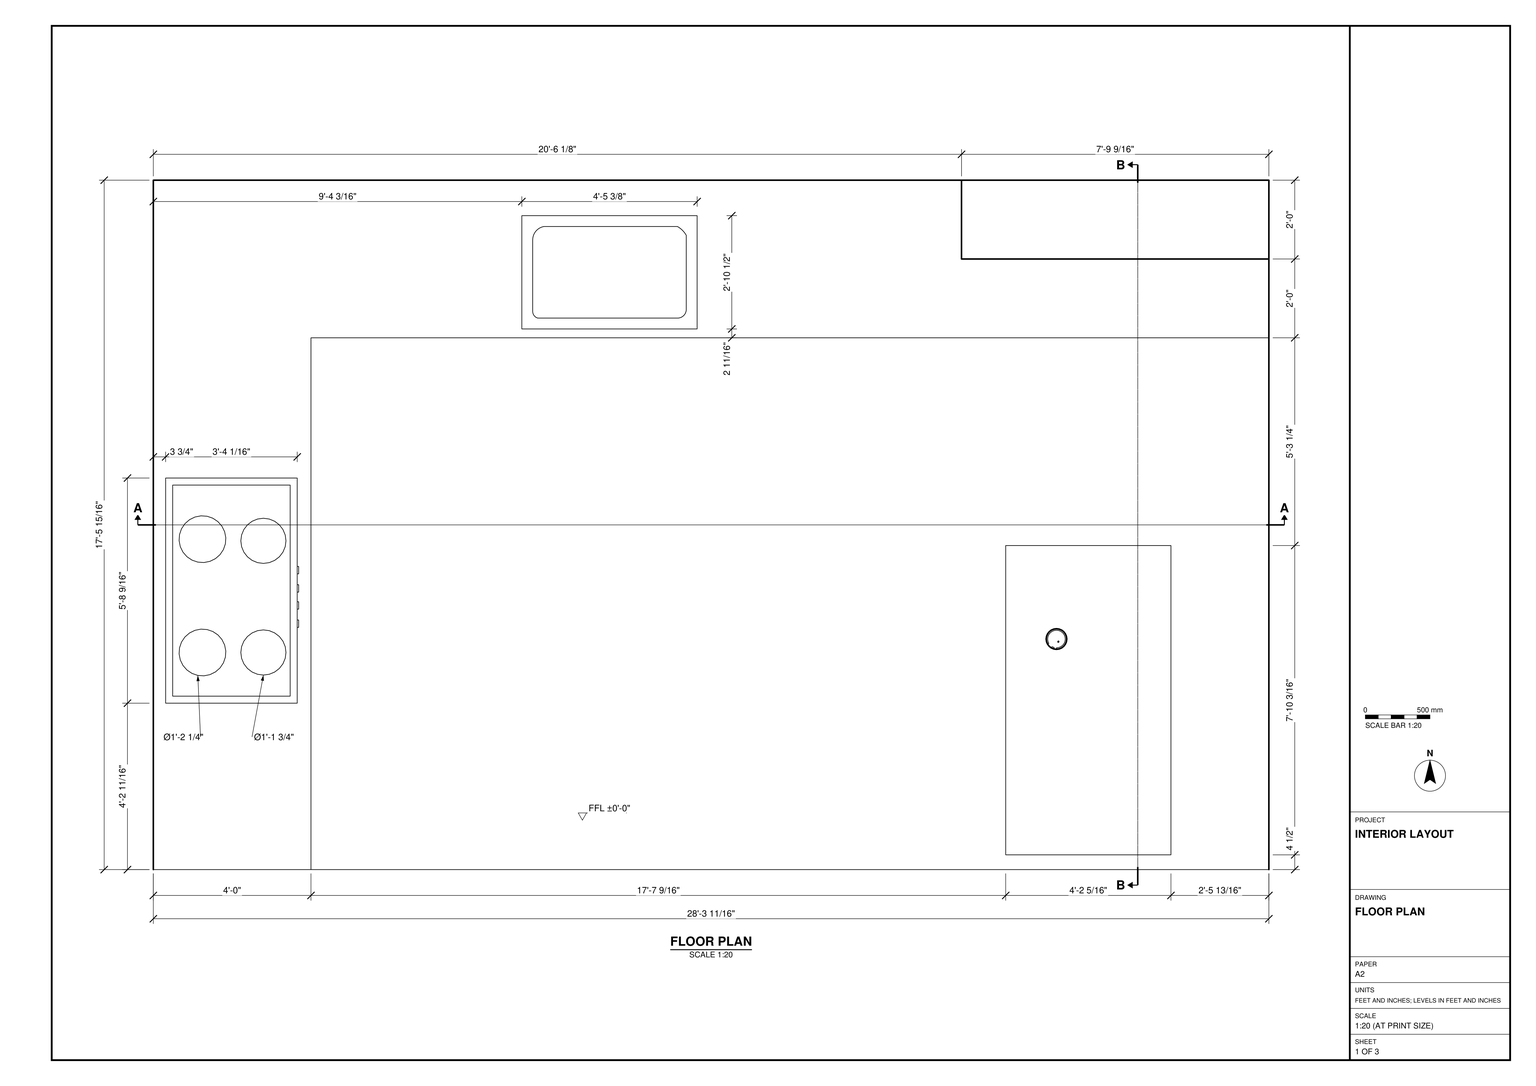
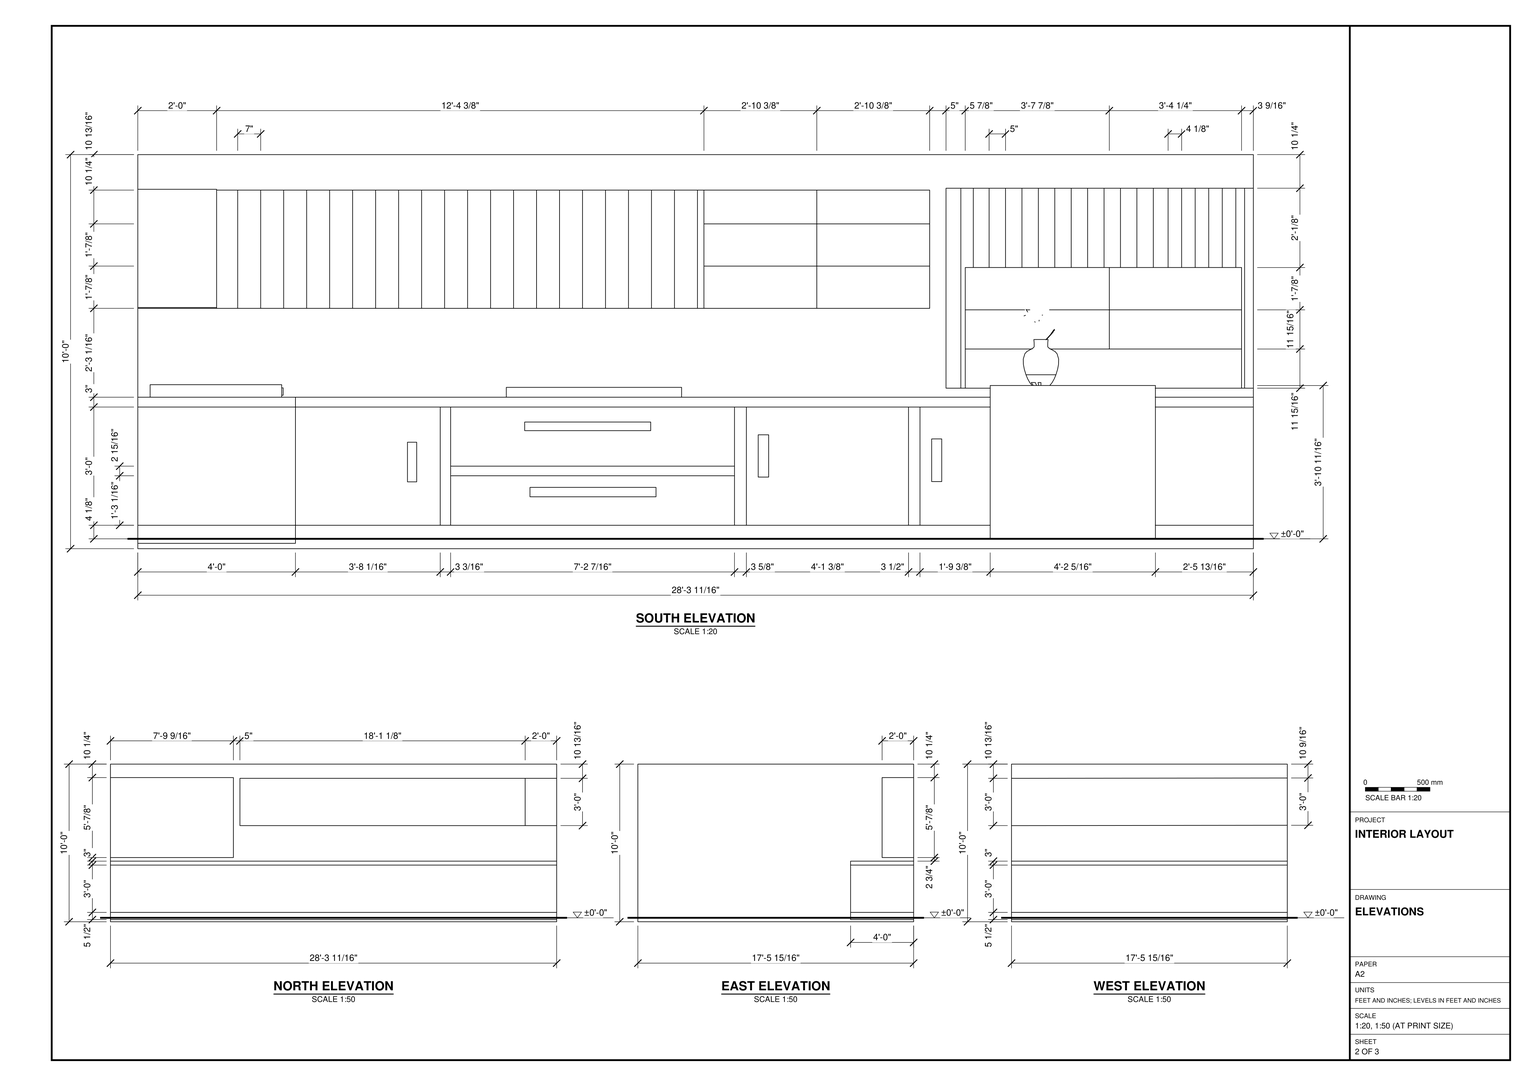
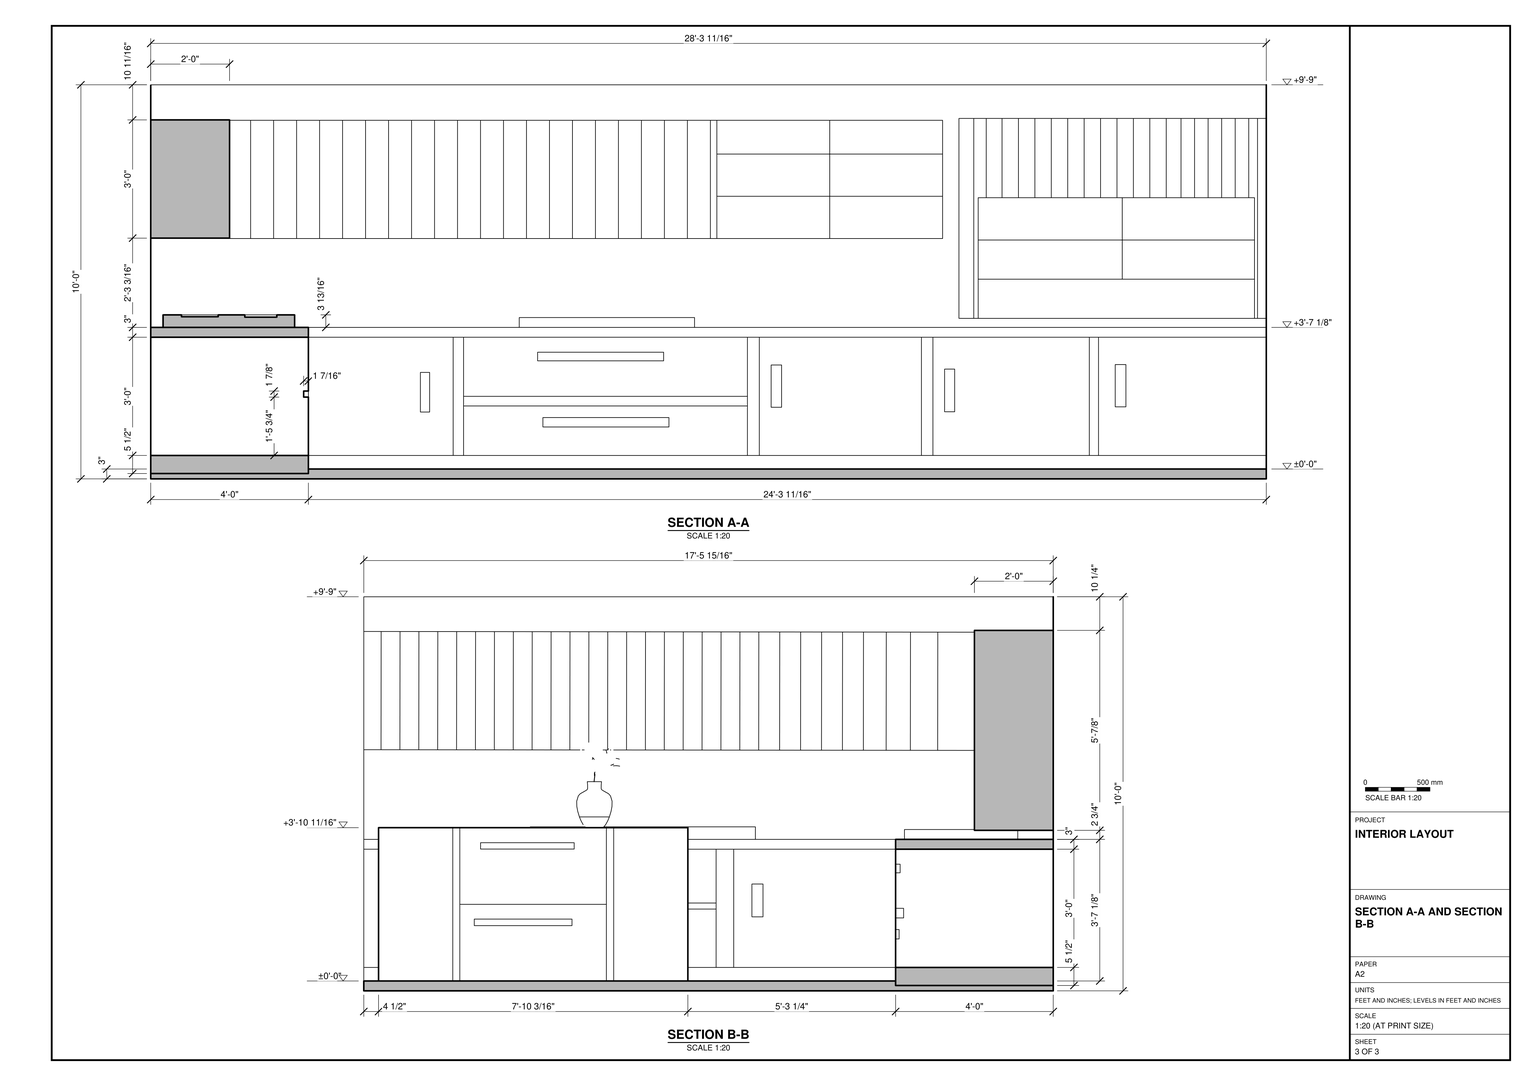
Build the kitchen interior in SketchUp from task_files/diagram_01.pdf. Work in feet and inches. The overall size is 28'-3 11/16" along X, 17'-5 15/16" along Y and 10'-0" vertically. Use the single finished-floor level of ±0'-0". Model the floor slab and the wall extents and thicknesses shown in the elevations and sections.

Use the floor plan to lay out the L-shaped counter along the top and left edges of the room. Place the sink in the long run and the cooktop on the left return. Use section A-A to set the worktop, plinth and cabinet heights. Match the arrangement of base cabinet doors, wide drawers and pulls. Above the worktop, distinguish the long band of narrow vertical panels from the horizontally divided cabinet bays, including the deeper hanging unit at the right end of the south elevation.

Set out the freestanding island from the bottom and right edges of the plan, with its long side parallel to the cooktop return. Use section B-B for its top height and drawer arrangement. Place a vase on the island as shown. Decor and loose items may be any suitable library components, for example from 3D Warehouse.

Keep shell elements such as walls and the floor slab in separate groups or components, group each furniture or joinery piece separately, and use components for repeated parts. Save one SketchUp model as output_files/l_shaped_kitchen_with_a_freestanding_storage_island.skp.

# SketchUp Ruby script. Lengths in inches.
U = 1.inch
M = Sketchup.active_model
def pt(a) = Geom::Point3d.new(a.map { |v| v * U })
def face(e, loops, mat)
  f = e.add_face(loops[0].map { |a| pt(a) })
  loops[1..].each { |l| e.add_face(l.map { |a| pt(a) }).erase! }
  f.material = f.back_material = mat if mat
  f
end
# faces: each face lists its corners as indices into pts; further lists are holes
def faces(e, pts, list, mat = nil) = list.each { |f| face(e, (f[0].is_a?(Array) ? f : [f]).map { |l| l.map { |i| pts[i] } }, mat) }
# xy, xz, yz: faces in a plane at the given z, y or x. An outline is a flat list of corners, or four numbers for a rectangle; further outlines are holes
def ring(l) = l.size == 4 ? [[l[0], l[1]], [l[2], l[1]], [l[2], l[3]], [l[0], l[3]]] : l.each_slice(2).to_a
def flat(e, list, mat, &to3) = list.each { |f| face(e, (f[0].is_a?(Array) ? f : [f]).map { |l| ring(l).map { |u, v| to3.(u, v) } }, mat) }
def xy(e, z, list, mat = nil) = flat(e, list, mat) { |x, y| [x, y, z] }
def xz(e, y, list, mat = nil) = flat(e, list, mat) { |x, z| [x, y, z] }
def yz(e, x, list, mat = nil) = flat(e, list, mat) { |y, z| [x, y, z] }
def lines(e, pts, list) = list.each { |a, b| e.add_line(pt(pts[a]), pt(pts[b])) }
# prism: a flat outline (further loops are holes) pulled along v
def prism(e, loops, v, mat = nil)
  f = face(e, loops, mat); d = Geom::Vector3d.new(v.map { |x| x * U })
  f.pushpull(f.normal.samedirection?(d) ? d.length : -d.length)
end
def box(e, o, s, mat = nil) = prism(e, [[o, [o[0] + s[0], o[1], o[2]], [o[0] + s[0], o[1] + s[1], o[2]], [o[0], o[1] + s[1], o[2]]]], [0, 0, s[2]], mat)
def at(x, y, z, deg = 0) = Geom::Transformation.translation(pt([x, y, z])) * Geom::Transformation.rotation(ORIGIN, Z_AXIS, deg.degrees)
def axes(o, x, y, z) = Geom::Transformation.new([*x, 0, *y, 0, *z, 0, *pt(o).to_a, 1])
def part(name) = M.definitions.add(name)
# library, detail: a bought-in or finely detailed component or shape, given as its bounding box
def library(name, o, s) = part(name).tap { |d| box(d.entities, o, s) }
def detail(e, o, s) = box(e.add_group.entities, o, s)
def put(e, d, t, mat = nil) = e.add_instance(d, t).tap { |i| i.material = mat if mat }
def group(e, t, mat = nil) = e.add_group.tap { |g| g.transformation = t; g.material = mat if mat }.entities
root = M.entities
M.materials.add("[Blacktop New]").color = [30, 30, 30]
M.materials.add("[Blacktop Old 01]").color = [132, 136, 139]
M.materials.add("[Blinds Weave]").color = [141, 91, 25]
M.materials.add("[Concrete Tile]").color = [203, 190, 164]
M.materials.add("[Tile Ceramic Natural]").color = [216, 206, 153]
M.materials.add("[Tile Limestone Multi]").color = [199, 173, 118]
M.materials.add("[Translucent Glass Block Dark]").color = [124, 124, 121]
M.materials["[Translucent Glass Block Dark]"].alpha = 0.8
M.materials.add("[Translucent Glass Blue]").color = [100, 149, 237]
M.materials["[Translucent Glass Blue]"].alpha = 0.5
c1 = library("Flower+vase",[-27.04,-0.0625,0],[7.8,7.11,11.89])
xy(root,0,[[0,0,339.6875,209.9375]])
xy(root,1.625,[[0,0,0,209.9375,339.6875,209.9375,339.6875,161.9375,48,161.9375,48,0]])
xy(root,3,[[[48,0,339.6875,161.9375],[259.55,4.49,309.86,98.68]],[259.55,4.49,309.86,98.68]],"[Tile Ceramic Natural]")
xy(root,7.125,[[0,0,0,209.9375,339.6875,209.9375,339.6875,161.9375,48,161.9375,48,0]])
xy(root,15.8,[[119.41,161.9375,157.79,163]],"[Blacktop Old 01]")
xy(root,17.51,[[46.625,57.29,48,85.85]],"[Blacktop Old 01]")
xy(root,18.67,[[119.41,161.9375,157.79,163]])
xy(root,19.85,[[259.55,33.64,260.43,63.39]],"[Tile Ceramic Natural]")
xy(root,20.58,[[46.625,57.29,48,85.85]])
xy(root,21.85,[[259.55,33.64,260.43,63.39]],"[Tile Ceramic Natural]")
xy(root,22.2,[[95.26,161.9375,181.69,164.375]],"[Blacktop New]")
xy(root,24.9,[[46.5625,41.5,48,107.28]],"[Blacktop New]")
xy(root,25.125,[[95.26,161.9375,181.69,164.375]])
xy(root,26.74,[[46.5625,41.5,48,107.28]])
xy(root,34.63,[[46.875,55.84,48,85.21]],"[Blacktop New]")
xy(root,35.94,[[117.8,161.9375,156.18,163.3125]],"[Blacktop New]")
xy(root,38.38,[[46.875,55.84,48,85.21]])
xy(root,38.57,[[117.8,161.9375,156.18,163.3125]])
xy(root,43.125,[[0,0,0,209.9375,339.6875,209.9375,339.6875,161.9375,48,161.9375,48,0]])
xy(root,43.17,[[259.55,35.5625,260.74,64.0625]],"[Tile Ceramic Natural]")
xy(root,45.11,[[259.55,35.5625,260.74,64.0625]],"[Tile Ceramic Natural]")
xy(root,46.125,[[[0,0,48,0,48,161.9375,339.6875,161.9375,339.6875,209.9375,0,209.9375],[3.75,50.67,43.8125,119.24],[112.21,164.64,165.59,199.14]],[3.75,50.67,43.8125,119.24],[[112.21,164.64,165.59,199.14],[117.08,167.94,159.625,167.94,159.97,167.96,160.3125,168.03,160.64,168.14,160.95,168.3,161.24,168.49,161.5,168.72,161.73,168.98,161.93,169.27,162.08,169.58,162.19,169.91,162.26,170.25,162.28,170.6,162.28,193.14,162.12,193.42,161.94,193.6875,161.75,193.95,161.55,194.2,161.34,194.4375,161.12,194.67,160.89,194.89,160.65,195.1,160.4,195.3,160.14,195.49,159.87,195.67,159.59,195.83,118.91,195.83,118.45,195.72,118,195.55,117.57,195.33,117.17,195.07,116.8,194.76,116.48,194.41,116.19,194.02,115.95,193.61,115.76,193.17,115.63,192.71,115.54,192.24,115.52,191.76,115.52,169.98,115.53,169.75,115.57,169.53,115.63,169.31,115.71,169.09,115.82,168.89,115.95,168.7,116.1,168.53,116.27,168.37,116.45,168.23,116.65,168.11,116.86,168.01]]],"[Concrete Tile]")
xy(root,48.875,[[246.09,185.9375,339.6875,209.9375]])
xy(root,49,[[33.51,59.24,35.29,59.48,36.95,60.16,38.375,61.26,39.47,62.68,40.15,64.34,40.39,66.12,40.15,67.9,39.47,69.56,38.375,70.98,36.95,72.07,35.29,72.76,33.51,72.99,31.73,72.76,30.08,72.07,28.65,70.98,27.56,69.56,26.875,67.9,26.64,66.12,26.875,64.34,27.56,62.68,28.65,61.26,30.08,60.16,31.73,59.48]],"[Concrete Tile]")
xy(root,49.125,[[[112.21,164.64,165.59,199.14],[117.08,167.94,116.86,168.01,116.65,168.11,116.45,168.23,116.27,168.37,116.1,168.53,115.95,168.7,115.82,168.89,115.71,169.09,115.63,169.31,115.57,169.53,115.53,169.75,115.52,169.98,115.52,191.76,115.54,192.24,115.63,192.71,115.76,193.17,115.95,193.61,116.19,194.02,116.48,194.41,116.8,194.76,117.17,195.07,117.57,195.33,118,195.55,118.45,195.72,118.91,195.83,159.59,195.83,159.87,195.67,160.14,195.49,160.4,195.3,160.65,195.1,160.89,194.89,161.12,194.67,161.34,194.4375,161.55,194.2,161.75,193.95,161.94,193.6875,162.12,193.42,162.28,193.14,162.28,170.6,162.26,170.25,162.19,169.91,162.08,169.58,161.93,169.27,161.73,168.98,161.5,168.72,161.24,168.49,160.95,168.3,160.64,168.14,160.3125,168.03,159.97,167.96,159.625,167.94]]],"[Concrete Tile]")
xy(root,49.25,[[33.51,93.24,35.29,93.48,36.95,94.16,38.375,95.26,39.47,96.68,40.15,98.34,40.39,100.12,40.15,101.9,39.47,103.56,38.375,104.98,36.95,106.07,35.29,106.76,33.51,106.99,31.73,106.76,30.08,106.07,28.65,104.98,27.56,103.56,26.875,101.9,26.64,100.12,26.875,98.34,27.56,96.68,28.65,95.26,30.08,94.16,31.73,93.48]],"[Concrete Tile]")
xy(root,49.375,[[15.41,59.01,17.23,59.37,18.9,60.1875,20.3,61.41,21.34,62.95,21.94,64.71,22.07,66.57,21.71,68.39,20.89,70.0625,19.67,71.47,18.12,72.5,16.36,73.1,14.5,73.23,12.68,72.87,11.01,72.05,9.61,70.83,8.57,69.28,7.97,67.52,7.85,65.67,8.2,63.84,9.02,62.17,10.25,60.77,11.79,59.73,13.55,59.13],[15.41,93.51,17.23,93.87,18.9,94.6875,20.3,95.91,21.34,97.45,21.94,99.21,22.07,101.07,21.71,102.89,20.89,104.5625,19.67,105.97,18.12,107,16.36,107.6,14.5,107.73,12.68,107.37,11.01,106.55,9.61,105.33,8.57,103.78,7.97,102.02,7.85,100.17,8.2,98.34,9.02,96.67,10.25,95.27,11.79,94.23,13.55,93.63]],"[Concrete Tile]")
xy(root,49.6875,[[259.55,4.49,309.86,98.68]],"[Tile Ceramic Natural]")
xy(root,49.9375,[[[5.89,52.81,41.67,117.09],[15.41,59.01,13.55,59.13,11.79,59.73,10.25,60.77,9.02,62.17,8.2,63.84,7.85,65.67,7.97,67.52,8.57,69.28,9.61,70.83,11.01,72.05,12.68,72.87,14.5,73.23,16.36,73.1,18.12,72.5,19.67,71.47,20.89,70.0625,21.71,68.39,22.07,66.57,21.94,64.71,21.34,62.95,20.3,61.41,18.9,60.1875,17.23,59.37],[15.41,93.51,13.55,93.63,11.79,94.23,10.25,95.27,9.02,96.67,8.2,98.34,7.85,100.17,7.97,102.02,8.57,103.78,9.61,105.33,11.01,106.55,12.68,107.37,14.5,107.73,16.36,107.6,18.12,107,19.67,105.97,20.89,104.5625,21.71,102.89,22.07,101.07,21.94,99.21,21.34,97.45,20.3,95.91,18.9,94.6875,17.23,93.87],[33.51,59.24,31.73,59.48,30.08,60.16,28.65,61.26,27.56,62.68,26.875,64.34,26.64,66.12,26.875,67.9,27.56,69.56,28.65,70.98,30.08,72.07,31.73,72.76,33.51,72.99,35.29,72.76,36.95,72.07,38.375,70.98,39.47,69.56,40.15,67.9,40.39,66.12,40.15,64.34,39.47,62.68,38.375,61.26,36.95,60.16,35.29,59.48],[33.51,93.24,31.73,93.48,30.08,94.16,28.65,95.26,27.56,96.68,26.875,98.34,26.64,100.12,26.875,101.9,27.56,103.56,28.65,104.98,30.08,106.07,31.73,106.76,33.51,106.99,35.29,106.76,36.95,106.07,38.375,104.98,39.47,103.56,40.15,101.9,40.39,100.12,40.15,98.34,39.47,96.68,38.375,95.26,36.95,94.16,35.29,93.48]]],"[Blacktop New]")
xy(root,49.9375,[[[3.75,50.67,43.8125,119.24],[5.89,52.81,41.67,117.09]]],"[Concrete Tile]")
xy(root,73.1875,[[24,185.9375,241.125,209.9375]],"[Blinds Weave]")
xy(root,109.1875,[[24,185.9375,241.125,209.9375]],"[Blinds Weave]")
xy(root,109.76,[[246.09,185.9375,339.6875,209.9375]],"[Blinds Weave]")
xz(root,0,[[0,73.4375,24,109.4375]],"[Blinds Weave]")
xz(root,0,[[0,43.125,48,46.125]],"[Concrete Tile]")
xz(root,0,[[0,0,339.6875,0,339.6875,3,48,3,48,1.625,0,1.625]],"[Tile Ceramic Natural]")
xz(root,0,[[0,1.625,48,7.125],[0,7.125,48,43.125]],"[Tile Limestone Multi]")
xz(root,4.49,[[259.55,3,309.86,49.6875]],"[Tile Ceramic Natural]")
xz(root,33.64,[[259.55,19.85,260.43,21.85]],"[Tile Ceramic Natural]")
xz(root,35.5625,[[259.55,43.17,260.74,45.11]],"[Tile Ceramic Natural]")
xz(root,41.5,[[46.5625,24.9,48,26.74]])
xz(root,50.67,[[3.75,46.125,43.8125,49.9375]],"[Concrete Tile]")
xz(root,55.84,[[46.875,34.63,48,38.38]])
xz(root,57.29,[[46.625,17.51,48,20.58]])
xz(root,63.39,[[259.55,19.85,260.43,21.85]],"[Tile Ceramic Natural]")
xz(root,64.0625,[[259.55,43.17,260.74,45.11]],"[Tile Ceramic Natural]")
xz(root,85.21,[[46.875,34.63,48,38.38]],"[Blacktop New]")
xz(root,85.85,[[46.625,17.51,48,20.58]],"[Blacktop Old 01]")
xz(root,98.68,[[259.55,3,309.86,49.6875]],"[Tile Ceramic Natural]")
xz(root,107.28,[[46.5625,24.9,48,26.74]],"[Blacktop Old 01]")
xz(root,119.24,[[3.75,46.125,43.8125,49.9375]],"[Concrete Tile]")
xz(root,161.9375,[[48,1.625,339.6875,3]])
xz(root,161.9375,[[82.11,20.35,84.92,32.42],[241.73,20.43,244.79,33.43],[188.91,21.8,192.1,34.68],[293.6875,21.93,296.9375,34.81]],"[Blacktop Old 01]")
xz(root,161.9375,[[48,43.125,339.6875,46.125]],"[Concrete Tile]")
xz(root,161.9375,[[48,3,339.6875,7.125],[[48,7.125,92.09,43.125],[82.11,20.35,84.92,32.42]],[92.09,7.125,95.26,43.125],[[95.26,7.125,181.69,22.2],[119.41,15.8,157.79,18.67]],[181.69,7.125,185.3125,43.125],
  [[185.3125,7.125,234.68,43.125],[188.91,21.8,192.1,34.68]],[234.68,7.125,238.18,43.125],[[238.18,7.125,285.8,43.125],[241.73,20.43,244.79,33.43]],[285.8,7.125,288.6,43.125],[[288.6,7.125,339.6875,43.125],[293.6875,21.93,296.9375,34.81]],
  [[95.26,25.125,181.69,43.125],[117.8,35.94,156.18,38.57]]],"[Tile Limestone Multi]")
xz(root,163,[[119.41,15.8,157.79,18.67]],"[Blacktop Old 01]")
xz(root,163.3125,[[117.8,35.94,156.18,38.57]],"[Blacktop New]")
xz(root,164.375,[[95.26,22.2,181.69,25.125]],"[Blacktop New]")
xz(root,164.64,[[112.21,46.125,165.59,49.125]],"[Concrete Tile]")
xz(root,167.94,[[117.08,46.125,159.625,49.125]],"[Concrete Tile]")
xz(root,185.9375,[[246.09,48.875,250.61,109.76],[250.61,48.875,251.96,48.875,251.96,85.62,254.41,85.62,254.41,109.76,250.61,109.76],[336.09,48.875,337.02,48.875,337.02,109.76,334.35,109.76,334.35,85.62,336.09,85.62],[337.02,48.875,339.6875,109.76],[24,73.1875,172.38,109.1875],
  [254.41,85.62,259.22,109.76],[259.22,85.62,264.22,109.76],[264.22,85.62,269.22,109.76],[269.22,85.62,274.22,109.76],[274.22,85.62,279.22,109.76],
  [279.22,85.62,284.22,109.76],[284.22,85.62,289.22,109.76],[289.22,85.62,294.22,109.76],[294.22,85.62,299.22,109.76],[299.22,85.62,304.22,109.76],
  [304.22,85.62,309.22,109.76],[309.22,85.62,313.72,109.76],[313.72,85.62,317.85,109.76],[317.85,85.62,321.97,109.76],[321.97,85.62,326.1,109.76],
  [326.1,85.62,330.22,109.76],[330.22,85.62,334.35,109.76]],"[Blinds Weave]")
xz(root,185.9375,[[251.96,48.875,336.09,60.8]],"[Translucent Glass Block Dark]")
xz(root,185.9375,[[251.96,60.8,295.82,72.73],[295.82,60.8,336.09,72.73],[251.96,72.73,295.82,85.62],[295.82,72.73,336.09,85.62],[172.38,73.1875,206.75,86.05],
  [206.75,73.1875,241.125,86.05],[172.38,86.05,206.75,98.91],[206.75,86.05,241.125,98.91],[172.38,98.91,206.75,109.1875],[206.75,98.91,241.125,109.1875]],"[Translucent Glass Blue]")
xz(root,195.83,[[118.91,46.125,159.59,49.125]],"[Concrete Tile]")
xz(root,199.14,[[112.21,46.125,165.59,49.125]],"[Concrete Tile]")
xz(root,209.9375,[[0,0,339.6875,1.625],[0,1.625,339.6875,7.125],[0,7.125,339.6875,43.125],[0,43.125,339.6875,46.125],[0,46.125,0,73.1875,241.125,73.1875,241.125,109.1875,0,109.1875,0,120,339.6875,120,339.6875,109.76,246.09,109.76,246.09,48.875,339.6875,48.875,339.6875,46.125],
  [246.09,48.875,339.6875,109.76],[0,73.1875,24,109.1875],[24,73.1875,241.125,109.1875]],"[Blacktop Old 01]")
yz(root,0,[[0,0,209.9375,1.625]])
yz(root,0,[[0,1.625,209.9375,7.125],[0,7.125,209.9375,43.125],[0,43.125,209.9375,46.125],[0,46.125,0,73.4375,209.9375,73.1875,209.9375,46.125],[209.9375,73.1875,0,73.4375,0,109.4375,209.9375,109.1875],
  [209.9375,109.1875,0,109.4375,0,120,209.9375,120]],"[Blacktop Old 01]")
yz(root,3.75,[[50.67,46.125,119.24,49.9375]],"[Concrete Tile]")
yz(root,24,[[185.9375,73.1875,185.9375,73.22,209.9375,73.1875],[209.9375,73.1875,209.9375,109.1875,185.9375,109.1875,185.9375,73.22]])
yz(root,24,[[185.9375,73.22,185.9375,109.1875,209.9375,109.1875,174.78,109.23,166.47,109.24,166.43,73.24],[166.43,73.24,166.47,109.24,159.1,109.25,159.05,73.25],[159.05,73.25,159.1,109.25,152.16,109.26,152.12,73.26],[145.74,73.26,145.78,109.26,139.41,109.27,139.37,73.27],[145.74,73.26,152.12,73.26,152.16,109.26,145.78,109.26],
  [139.37,73.27,139.41,109.27,133.03,109.28,132.99,73.28],[132.99,73.28,133.03,109.28,126.66,109.29,126.62,73.29],[120.24,73.29,120.28,109.29,114.53,109.3,114.49,73.3],[120.24,73.29,126.62,73.29,126.66,109.29,120.28,109.29],[114.49,73.3,114.53,109.3,108.78,109.31,108.74,73.31],
  [102.99,73.31,103.03,109.31,97.28,109.32,97.24,73.32],[102.99,73.31,108.74,73.31,108.78,109.31,103.03,109.31],[97.24,73.32,97.28,109.32,91.53,109.33,91.49,73.33],[91.49,73.33,91.53,109.33,85.78,109.34,85.74,73.34],[79.99,73.34,80.03,109.34,74.28,109.35,74.24,73.35],
  [79.99,73.34,85.74,73.34,85.78,109.34,80.03,109.34],[74.24,73.35,74.28,109.35,68.53,109.36,68.49,73.36],[62.74,73.36,62.78,109.36,57.03,109.37,56.99,73.37],[62.74,73.36,68.49,73.36,68.53,109.36,62.78,109.36],[56.99,73.37,57.03,109.37,51.28,109.375,51.24,73.375],
  [51.24,73.375,51.28,109.375,45.53,109.38,45.49,73.38],[45.49,73.38,45.53,109.38,39.79,109.39,39.74,73.39],[39.74,73.39,39.79,109.39,34.04,109.4,33.99,73.4],[28.24,73.4,28.29,109.4,22.54,109.41,22.49,73.41],[28.24,73.4,33.99,73.4,34.04,109.4,28.29,109.4],
  [22.49,73.41,22.54,109.41,16.79,109.42,16.74,73.42],[10.99,73.42,11.04,109.42,5.29,109.43,5.24,73.43],[10.99,73.42,16.74,73.42,16.79,109.42,11.04,109.42],[5.24,73.43,5.29,109.43,0,109.4375,0,73.4375]],"[Blinds Weave]")
yz(root,43.8125,[[[50.67,46.125,119.24,49.9375],[74.875,46.72,74.59,46.76,74.3125,46.87,74.08,47.05,73.9,47.28,73.79,47.55,73.75,47.85,73.79,48.14,73.9,48.41,74.08,48.64,74.3125,48.82,74.59,48.93,74.875,48.97,75.17,48.93,75.4375,48.82,75.67,48.64,75.85,48.41,75.96,48.14,76,47.85,75.96,47.55,75.85,47.28,75.67,47.05,75.4375,46.87,75.17,46.76],[80.4375,46.72,80.15,46.76,79.875,46.87,79.64,47.05,79.46,47.28,79.35,47.55,79.3125,47.85,79.35,48.14,79.46,48.41,79.64,48.64,79.875,48.82,80.15,48.93,80.4375,48.97,80.73,48.93,81,48.82,81.23,48.64,81.41,48.41,81.53,48.14,81.5625,47.85,81.53,47.55,81.41,47.28,81.23,47.05,81,46.87,80.73,46.76],[91.1875,46.72,90.9,46.76,90.625,46.87,90.39,47.05,90.21,47.28,90.1,47.55,90.0625,47.85,90.1,48.14,90.21,48.41,90.39,48.64,90.625,48.82,90.9,48.93,91.1875,48.97,91.48,48.93,91.75,48.82,91.98,48.64,92.16,48.41,92.28,48.14,92.3125,47.85,92.28,47.55,92.16,47.28,91.98,47.05,91.75,46.87,91.48,46.76],[85.625,46.72,85.34,46.76,85.0625,46.87,84.83,47.05,84.65,47.28,84.54,47.55,84.5,47.85,84.54,48.14,84.65,48.41,84.83,48.64,85.0625,48.82,85.34,48.93,85.625,48.97,85.92,48.93,86.1875,48.82,86.42,48.64,86.6,48.41,86.71,48.14,86.75,47.85,86.71,47.55,86.6,47.28,86.42,47.05,86.1875,46.87,85.92,46.76]]],"[Blacktop New]")
yz(root,43.8125,[[74.875,46.72,74.59,46.76,74.3125,46.87,74.08,47.05,73.9,47.28,73.79,47.55,73.75,47.85,73.79,48.14,73.9,48.41,74.08,48.64,74.3125,48.82,74.59,48.93,74.875,48.97,75.17,48.93,75.4375,48.82,75.67,48.64,75.85,48.41,75.96,48.14,76,47.85,75.96,47.55,75.85,47.28,75.67,47.05,75.4375,46.87,75.17,46.76],[80.4375,46.72,80.15,46.76,79.875,46.87,79.64,47.05,79.46,47.28,79.35,47.55,79.3125,47.85,79.35,48.14,79.46,48.41,79.64,48.64,79.875,48.82,80.15,48.93,80.4375,48.97,80.73,48.93,81,48.82,81.23,48.64,81.41,48.41,81.53,48.14,81.5625,47.85,81.53,47.55,81.41,47.28,81.23,47.05,81,46.87,80.73,46.76],[85.625,46.72,85.34,46.76,85.0625,46.87,84.83,47.05,84.65,47.28,84.54,47.55,84.5,47.85,84.54,48.14,84.65,48.41,84.83,48.64,85.0625,48.82,85.34,48.93,85.625,48.97,85.92,48.93,86.1875,48.82,86.42,48.64,86.6,48.41,86.71,48.14,86.75,47.85,86.71,47.55,86.6,47.28,86.42,47.05,86.1875,46.87,85.92,46.76],[91.1875,46.72,90.9,46.76,90.625,46.87,90.39,47.05,90.21,47.28,90.1,47.55,90.0625,47.85,90.1,48.14,90.21,48.41,90.39,48.64,90.625,48.82,90.9,48.93,91.1875,48.97,91.48,48.93,91.75,48.82,91.98,48.64,92.16,48.41,92.28,48.14,92.3125,47.85,92.28,47.55,92.16,47.28,91.98,47.05,91.75,46.87,91.48,46.76]],"[Concrete Tile]")
yz(root,44.25,[[74.875,46.72,75.17,46.76,75.4375,46.87,75.67,47.05,75.85,47.28,75.96,47.55,76,47.85,75.96,48.14,75.85,48.41,75.67,48.64,75.4375,48.82,75.17,48.93,74.875,48.97,74.59,48.93,74.3125,48.82,74.08,48.64,73.9,48.41,73.79,48.14,73.75,47.85,73.79,47.55,73.9,47.28,74.08,47.05,74.3125,46.87,74.59,46.76],[80.4375,46.72,80.73,46.76,81,46.87,81.23,47.05,81.41,47.28,81.53,47.55,81.5625,47.85,81.53,48.14,81.41,48.41,81.23,48.64,81,48.82,80.73,48.93,80.4375,48.97,80.15,48.93,79.875,48.82,79.64,48.64,79.46,48.41,79.35,48.14,79.3125,47.85,79.35,47.55,79.46,47.28,79.64,47.05,79.875,46.87,80.15,46.76],[85.625,46.72,85.92,46.76,86.1875,46.87,86.42,47.05,86.6,47.28,86.71,47.55,86.75,47.85,86.71,48.14,86.6,48.41,86.42,48.64,86.1875,48.82,85.92,48.93,85.625,48.97,85.34,48.93,85.0625,48.82,84.83,48.64,84.65,48.41,84.54,48.14,84.5,47.85,84.54,47.55,84.65,47.28,84.83,47.05,85.0625,46.87,85.34,46.76],[91.1875,46.72,91.48,46.76,91.75,46.87,91.98,47.05,92.16,47.28,92.28,47.55,92.3125,47.85,92.28,48.14,92.16,48.41,91.98,48.64,91.75,48.82,91.48,48.93,91.1875,48.97,90.9,48.93,90.625,48.82,90.39,48.64,90.21,48.41,90.1,48.14,90.0625,47.85,90.1,47.55,90.21,47.28,90.39,47.05,90.625,46.87,90.9,46.76]],"[Concrete Tile]")
yz(root,46.5625,[[41.5,24.9,107.28,26.74]],"[Blacktop New]")
yz(root,46.625,[[57.29,17.51,85.85,20.58]],"[Blacktop Old 01]")
yz(root,46.875,[[55.84,34.63,85.21,38.38]],"[Blacktop New]")
yz(root,48,[[0,1.625,161.9375,3]])
yz(root,48,[[118.1875,22.53,121.5625,32.53],[29.1,22.67,31.85,33.42]],"[Blacktop Old 01]")
yz(root,48,[[0,43.125,161.9375,46.125]],"[Concrete Tile]")
yz(root,48,[[0,3,161.9375,7.125],[[0,7.125,37.12,43.125],[29.1,22.67,31.85,33.42]],[37.12,7.125,41.5,43.125],[[41.5,7.125,107.28,24.9],[57.29,17.51,85.85,20.58]],[107.28,7.125,112.64,43.125],
  [[112.64,7.125,161.9375,43.125],[118.1875,22.53,121.5625,32.53]],[[41.5,26.74,107.28,43.125],[55.84,34.63,85.21,38.38]]],"[Tile Limestone Multi]")
yz(root,95.26,[[161.9375,22.2,164.375,25.125]],"[Blacktop New]")
yz(root,112.21,[[164.64,46.125,199.14,49.125]],"[Concrete Tile]")
yz(root,115.52,[[169.98,46.125,191.76,49.125]],"[Concrete Tile]")
yz(root,117.8,[[161.9375,35.94,163.3125,38.57]],"[Blacktop New]")
yz(root,119.41,[[161.9375,15.8,163,18.67]])
yz(root,156.18,[[161.9375,35.94,163.3125,38.57]],"[Blacktop New]")
yz(root,157.79,[[161.9375,15.8,163,18.67]])
yz(root,162.28,[[170.6,46.125,193.14,49.125]],"[Concrete Tile]")
yz(root,165.59,[[164.64,46.125,199.14,49.125]],"[Concrete Tile]")
yz(root,181.69,[[161.9375,22.2,164.375,25.125]],"[Blacktop New]")
yz(root,241.125,[[185.9375,73.1875,209.9375,109.1875]],"[Blinds Weave]")
yz(root,246.09,[[185.9375,48.875,209.9375,109.76]],"[Blinds Weave]")
yz(root,259.55,[[4.49,3,27.09,49.6875],[27.09,3,29.23,49.6875],[[29.23,3,73.86,26.34],[33.64,19.85,63.39,21.85]],[73.86,3,76.1,49.6875],[76.1,3,98.68,49.6875],
  [[29.23,26.34,73.86,49.6875],[35.5625,43.17,64.0625,45.11]]],"[Tile Ceramic Natural]")
yz(root,260.43,[[33.64,19.85,63.39,21.85]],"[Tile Ceramic Natural]")
yz(root,260.74,[[35.5625,43.17,64.0625,45.11]],"[Tile Ceramic Natural]")
yz(root,309.86,[[4.49,3,98.68,49.6875]],"[Tile Ceramic Natural]")
yz(root,339.6875,[[0,0,209.9375,0,209.9375,1.625,161.9375,1.625,161.9375,3,0,3],[161.9375,1.625,209.9375,7.125],[0,3,161.9375,3,161.9375,46.125,209.9375,46.125,209.9375,48.875,185.9375,48.875,185.9375,109.76,209.9375,109.76,209.9375,120,0,120],[161.9375,7.125,209.9375,43.125],[161.9375,43.125,209.9375,46.125],
  [185.9375,48.875,209.9375,109.76]],"[Blacktop Old 01]")
p = [[117.08,167.94,46.125],[116.86,168.01,46.125],[116.86,168.01,49.125],[117.08,167.94,49.125],[159.97,167.96,46.125],[159.625,167.94,46.125],
  [159.625,167.94,49.125],[159.97,167.96,49.125],[116.65,168.11,46.125],[116.65,168.11,49.125],[160.3125,168.03,46.125],[160.3125,168.03,49.125],
  [160.64,168.14,46.125],[160.64,168.14,49.125],[116.45,168.23,46.125],[116.45,168.23,49.125],[160.95,168.3,46.125],[160.95,168.3,49.125],
  [116.27,168.37,46.125],[116.27,168.37,49.125],[161.24,168.49,46.125],[161.24,168.49,49.125],[116.1,168.53,46.125],[116.1,168.53,49.125],
  [115.95,168.7,46.125],[115.95,168.7,49.125],[161.5,168.72,46.125],[161.5,168.72,49.125],[115.82,168.89,46.125],[115.82,168.89,49.125],
  [161.73,168.98,46.125],[161.73,168.98,49.125],[115.71,169.09,46.125],[115.71,169.09,49.125],[161.93,169.27,46.125],[161.93,169.27,49.125],
  [115.63,169.31,46.125],[115.63,169.31,49.125],[115.57,169.53,46.125],[115.57,169.53,49.125],[162.08,169.58,46.125],[162.08,169.58,49.125],
  [115.53,169.75,46.125],[115.53,169.75,49.125],[162.19,169.91,46.125],[162.19,169.91,49.125],[115.52,169.98,46.125],[115.52,169.98,49.125],
  [162.26,170.25,46.125],[162.26,170.25,49.125],[162.28,170.6,46.125],[162.28,170.6,49.125],[115.52,191.76,46.125],[115.54,192.24,46.125],
  [115.54,192.24,49.125],[115.52,191.76,49.125],[115.63,192.71,46.125],[115.63,192.71,49.125],[115.76,193.17,46.125],[115.76,193.17,49.125],
  [162.12,193.42,46.125],[162.28,193.14,46.125],[162.28,193.14,49.125],[162.12,193.42,49.125],[115.95,193.61,46.125],[115.95,193.61,49.125],
  [161.94,193.6875,46.125],[161.94,193.6875,49.125],[116.19,194.02,46.125],[116.19,194.02,49.125],[161.75,193.95,46.125],[161.75,193.95,49.125],
  [161.55,194.2,46.125],[161.55,194.2,49.125],[116.48,194.41,46.125],[116.48,194.41,49.125],[161.34,194.4375,46.125],[161.34,194.4375,49.125],
  [116.8,194.76,46.125],[116.8,194.76,49.125],[161.12,194.67,46.125],[161.12,194.67,49.125],[160.89,194.89,46.125],[160.89,194.89,49.125],
  [117.17,195.07,46.125],[117.17,195.07,49.125],[160.65,195.1,46.125],[160.65,195.1,49.125],[117.57,195.33,46.125],[117.57,195.33,49.125],
  [160.4,195.3,46.125],[160.4,195.3,49.125],[118,195.55,46.125],[118,195.55,49.125],[160.14,195.49,46.125],[160.14,195.49,49.125],
  [159.87,195.67,46.125],[159.87,195.67,49.125],[118.45,195.72,46.125],[118.45,195.72,49.125],[118.91,195.83,46.125],[118.91,195.83,49.125],
  [159.59,195.83,46.125],[159.59,195.83,49.125],[43.8125,74.59,46.76],[43.8125,74.875,46.72],[44.25,74.875,46.72],[44.25,74.59,46.76],
  [43.8125,75.17,46.76],[44.25,75.17,46.76],[43.8125,80.15,46.76],[43.8125,80.4375,46.72],[44.25,80.4375,46.72],[44.25,80.15,46.76],
  [43.8125,80.73,46.76],[44.25,80.73,46.76],[43.8125,85.34,46.76],[43.8125,85.625,46.72],[44.25,85.625,46.72],[44.25,85.34,46.76],
  [43.8125,85.92,46.76],[44.25,85.92,46.76],[43.8125,90.9,46.76],[43.8125,91.1875,46.72],[44.25,91.1875,46.72],[44.25,90.9,46.76],
  [43.8125,91.48,46.76],[44.25,91.48,46.76],[43.8125,74.3125,46.87],[44.25,74.3125,46.87],[43.8125,75.4375,46.87],[44.25,75.4375,46.87],
  [43.8125,79.875,46.87],[44.25,79.875,46.87],[43.8125,81,46.87],[44.25,81,46.87],[43.8125,85.0625,46.87],[44.25,85.0625,46.87],
  [43.8125,86.1875,46.87],[44.25,86.1875,46.87],[43.8125,90.625,46.87],[44.25,90.625,46.87],[43.8125,91.75,46.87],[44.25,91.75,46.87],
  [43.8125,74.08,47.05],[44.25,74.08,47.05],[43.8125,75.67,47.05],[44.25,75.67,47.05],[43.8125,79.64,47.05],[44.25,79.64,47.05],
  [43.8125,81.23,47.05],[44.25,81.23,47.05],[43.8125,84.83,47.05],[44.25,84.83,47.05],[43.8125,86.42,47.05],[44.25,86.42,47.05],
  [43.8125,90.39,47.05],[44.25,90.39,47.05],[43.8125,91.98,47.05],[44.25,91.98,47.05],[43.8125,73.9,47.28],[44.25,73.9,47.28],
  [43.8125,75.85,47.28],[44.25,75.85,47.28],[43.8125,79.46,47.28],[44.25,79.46,47.28],[43.8125,81.41,47.28],[44.25,81.41,47.28],
  [43.8125,84.65,47.28],[44.25,84.65,47.28],[43.8125,86.6,47.28],[44.25,86.6,47.28],[43.8125,90.21,47.28],[44.25,90.21,47.28],
  [43.8125,92.16,47.28],[44.25,92.16,47.28],[43.8125,73.79,47.55],[44.25,73.79,47.55],[43.8125,75.96,47.55],[44.25,75.96,47.55],
  [43.8125,79.35,47.55],[44.25,79.35,47.55],[43.8125,81.53,47.55],[44.25,81.53,47.55],[43.8125,84.54,47.55],[44.25,84.54,47.55],
  [43.8125,86.71,47.55],[44.25,86.71,47.55],[43.8125,90.1,47.55],[44.25,90.1,47.55],[43.8125,92.28,47.55],[44.25,92.28,47.55],
  [43.8125,73.75,47.85],[44.25,73.75,47.85],[43.8125,76,47.85],[44.25,76,47.85],[43.8125,79.3125,47.85],[44.25,79.3125,47.85],
  [43.8125,81.5625,47.85],[44.25,81.5625,47.85],[43.8125,84.5,47.85],[44.25,84.5,47.85],[43.8125,86.75,47.85],[44.25,86.75,47.85],
  [43.8125,90.0625,47.85],[44.25,90.0625,47.85],[43.8125,92.3125,47.85],[44.25,92.3125,47.85],[43.8125,73.79,48.14],[44.25,73.79,48.14],
  [43.8125,75.96,48.14],[44.25,75.96,48.14],[43.8125,79.35,48.14],[44.25,79.35,48.14],[43.8125,81.53,48.14],[44.25,81.53,48.14],
  [43.8125,84.54,48.14],[44.25,84.54,48.14],[43.8125,86.71,48.14],[44.25,86.71,48.14],[43.8125,90.1,48.14],[44.25,90.1,48.14],
  [43.8125,92.28,48.14],[44.25,92.28,48.14],[43.8125,73.9,48.41],[44.25,73.9,48.41],[43.8125,75.85,48.41],[44.25,75.85,48.41],
  [43.8125,79.46,48.41],[44.25,79.46,48.41],[43.8125,81.41,48.41],[44.25,81.41,48.41],[43.8125,84.65,48.41],[44.25,84.65,48.41],
  [43.8125,86.6,48.41],[44.25,86.6,48.41],[43.8125,90.21,48.41],[44.25,90.21,48.41],[43.8125,92.16,48.41],[44.25,92.16,48.41],
  [43.8125,74.08,48.64],[44.25,74.08,48.64],[43.8125,75.67,48.64],[44.25,75.67,48.64],[43.8125,79.64,48.64],[44.25,79.64,48.64],
  [43.8125,81.23,48.64],[44.25,81.23,48.64],[43.8125,84.83,48.64],[44.25,84.83,48.64],[43.8125,86.42,48.64],[44.25,86.42,48.64],
  [43.8125,90.39,48.64],[44.25,90.39,48.64],[43.8125,91.98,48.64],[44.25,91.98,48.64],[43.8125,74.3125,48.82],[44.25,74.3125,48.82],
  [43.8125,75.4375,48.82],[44.25,75.4375,48.82],[43.8125,79.875,48.82],[44.25,79.875,48.82],[43.8125,81,48.82],[44.25,81,48.82],
  [43.8125,85.0625,48.82],[44.25,85.0625,48.82],[43.8125,86.1875,48.82],[44.25,86.1875,48.82],[43.8125,90.625,48.82],[44.25,90.625,48.82],
  [43.8125,91.75,48.82],[44.25,91.75,48.82],[43.8125,74.59,48.93],[44.25,74.59,48.93],[43.8125,75.17,48.93],[44.25,75.17,48.93],
  [43.8125,80.15,48.93],[44.25,80.15,48.93],[43.8125,80.73,48.93],[44.25,80.73,48.93],[43.8125,85.34,48.93],[44.25,85.34,48.93],
  [43.8125,85.92,48.93],[44.25,85.92,48.93],[43.8125,90.9,48.93],[44.25,90.9,48.93],[43.8125,91.48,48.93],[44.25,91.48,48.93],
  [43.8125,74.875,48.97],[44.25,74.875,48.97],[43.8125,80.4375,48.97],[44.25,80.4375,48.97],[43.8125,85.625,48.97],[44.25,85.625,48.97],
  [43.8125,91.1875,48.97],[44.25,91.1875,48.97],[31.73,59.48,49.9375],[33.51,59.24,49.9375],[33.51,59.24,49],[31.73,59.48,49],
  [35.29,59.48,49.9375],[35.29,59.48,49],[30.08,60.16,49.9375],[30.08,60.16,49],[36.95,60.16,49.9375],[36.95,60.16,49],
  [28.65,61.26,49.9375],[28.65,61.26,49],[38.375,61.26,49.9375],[38.375,61.26,49],[27.56,62.68,49.9375],[27.56,62.68,49],
  [39.47,62.68,49.9375],[39.47,62.68,49],[26.875,64.34,49.9375],[26.875,64.34,49],[40.15,64.34,49.9375],[40.15,64.34,49],
  [26.64,66.12,49.9375],[26.64,66.12,49],[40.39,66.12,49.9375],[40.39,66.12,49],[26.875,67.9,49.9375],[26.875,67.9,49],
  [40.15,67.9,49.9375],[40.15,67.9,49],[27.56,69.56,49.9375],[27.56,69.56,49],[39.47,69.56,49.9375],[39.47,69.56,49],
  [28.65,70.98,49.9375],[28.65,70.98,49],[38.375,70.98,49.9375],[38.375,70.98,49],[30.08,72.07,49.9375],[30.08,72.07,49],
  [36.95,72.07,49.9375],[36.95,72.07,49],[31.73,72.76,49.9375],[31.73,72.76,49],[35.29,72.76,49.9375],[35.29,72.76,49],
  [33.51,72.99,49.9375],[33.51,72.99,49],[31.73,93.48,49.9375],[33.51,93.24,49.9375],[33.51,93.24,49.25],[31.73,93.48,49.25],
  [35.29,93.48,49.9375],[35.29,93.48,49.25],[30.08,94.16,49.9375],[30.08,94.16,49.25],[36.95,94.16,49.9375],[36.95,94.16,49.25],
  [28.65,95.26,49.9375],[28.65,95.26,49.25],[38.375,95.26,49.9375],[38.375,95.26,49.25],[27.56,96.68,49.9375],[27.56,96.68,49.25],
  [39.47,96.68,49.9375],[39.47,96.68,49.25],[26.875,98.34,49.9375],[26.875,98.34,49.25],[40.15,98.34,49.9375],[40.15,98.34,49.25],
  [26.64,100.12,49.9375],[26.64,100.12,49.25],[40.39,100.12,49.9375],[40.39,100.12,49.25],[26.875,101.9,49.9375],[26.875,101.9,49.25],
  [40.15,101.9,49.9375],[40.15,101.9,49.25],[27.56,103.56,49.9375],[27.56,103.56,49.25],[39.47,103.56,49.9375],[39.47,103.56,49.25],
  [28.65,104.98,49.9375],[28.65,104.98,49.25],[38.375,104.98,49.9375],[38.375,104.98,49.25],[30.08,106.07,49.9375],[30.08,106.07,49.25],
  [36.95,106.07,49.9375],[36.95,106.07,49.25],[31.73,106.76,49.9375],[31.73,106.76,49.25],[35.29,106.76,49.9375],[35.29,106.76,49.25],
  [33.51,106.99,49.9375],[33.51,106.99,49.25],[13.55,59.13,49.9375],[15.41,59.01,49.9375],[15.41,59.01,49.375],[13.55,59.13,49.375],
  [17.23,59.37,49.9375],[17.23,59.37,49.375],[11.79,59.73,49.9375],[11.79,59.73,49.375],[18.9,60.1875,49.9375],[18.9,60.1875,49.375],
  [10.25,60.77,49.9375],[10.25,60.77,49.375],[20.3,61.41,49.9375],[20.3,61.41,49.375],[9.02,62.17,49.9375],[9.02,62.17,49.375],
  [21.34,62.95,49.9375],[21.34,62.95,49.375],[8.2,63.84,49.9375],[8.2,63.84,49.375],[21.94,64.71,49.9375],[21.94,64.71,49.375],
  [7.85,65.67,49.9375],[7.85,65.67,49.375],[22.07,66.57,49.9375],[22.07,66.57,49.375],[7.97,67.52,49.9375],[7.97,67.52,49.375],
  [21.71,68.39,49.9375],[21.71,68.39,49.375],[8.57,69.28,49.9375],[8.57,69.28,49.375],[20.89,70.0625,49.9375],[20.89,70.0625,49.375],
  [9.61,70.83,49.9375],[9.61,70.83,49.375],[19.67,71.47,49.9375],[19.67,71.47,49.375],[11.01,72.05,49.9375],[11.01,72.05,49.375],
  [18.12,72.5,49.9375],[18.12,72.5,49.375],[12.68,72.87,49.9375],[12.68,72.87,49.375],[16.36,73.1,49.9375],[16.36,73.1,49.375],
  [14.5,73.23,49.9375],[14.5,73.23,49.375],[13.55,93.63,49.9375],[15.41,93.51,49.9375],[15.41,93.51,49.375],[13.55,93.63,49.375],
  [17.23,93.87,49.9375],[17.23,93.87,49.375],[11.79,94.23,49.9375],[11.79,94.23,49.375],[18.9,94.6875,49.9375],[18.9,94.6875,49.375],
  [10.25,95.27,49.9375],[10.25,95.27,49.375],[20.3,95.91,49.9375],[20.3,95.91,49.375],[9.02,96.67,49.9375],[9.02,96.67,49.375],
  [21.34,97.45,49.9375],[21.34,97.45,49.375],[8.2,98.34,49.9375],[8.2,98.34,49.375],[21.94,99.21,49.9375],[21.94,99.21,49.375],
  [7.85,100.17,49.9375],[7.85,100.17,49.375],[22.07,101.07,49.9375],[22.07,101.07,49.375],[7.97,102.02,49.9375],[7.97,102.02,49.375],
  [21.71,102.89,49.9375],[21.71,102.89,49.375],[8.57,103.78,49.9375],[8.57,103.78,49.375],[20.89,104.5625,49.9375],[20.89,104.5625,49.375],
  [9.61,105.33,49.9375],[9.61,105.33,49.375],[19.67,105.97,49.9375],[19.67,105.97,49.375],[11.01,106.55,49.9375],[11.01,106.55,49.375],
  [18.12,107,49.9375],[18.12,107,49.375],[12.68,107.37,49.9375],[12.68,107.37,49.375],[16.36,107.6,49.9375],[16.36,107.6,49.375],
  [14.5,107.73,49.9375],[14.5,107.73,49.375],[0,0,73.4375],[0,209.9375,73.1875],[24,209.9375,73.1875],[24,185.9375,73.22],
  [24,166.43,73.24],[24,159.05,73.25],[24,152.12,73.26],[24,145.74,73.26],[24,139.37,73.27],[24,132.99,73.28],
  [24,126.62,73.29],[24,120.24,73.29],[24,114.49,73.3],[24,108.74,73.31],[24,102.99,73.31],[24,97.24,73.32],
  [24,91.49,73.33],[24,85.74,73.34],[24,79.99,73.34],[24,74.24,73.35],[24,68.49,73.36],[24,62.74,73.36],
  [24,56.99,73.37],[24,51.24,73.375],[24,45.49,73.38],[24,39.74,73.39],[24,33.99,73.4],[24,28.24,73.4],
  [24,22.49,73.41],[24,16.74,73.42],[24,10.99,73.42],[24,5.24,73.43],[24,0,73.4375],[0,209.9375,109.1875],
  [0,0,109.4375],[24,0,109.4375],[24,5.29,109.43],[24,11.04,109.42],[24,16.79,109.42],[24,22.54,109.41],
  [24,28.29,109.4],[24,34.04,109.4],[24,39.79,109.39],[24,45.53,109.38],[24,51.28,109.375],[24,57.03,109.37],
  [24,62.78,109.36],[24,68.53,109.36],[24,74.28,109.35],[24,80.03,109.34],[24,85.78,109.34],[24,91.53,109.33],
  [24,97.28,109.32],[24,103.03,109.31],[24,108.78,109.31],[24,114.53,109.3],[24,120.28,109.29],[24,126.66,109.29],
  [24,133.03,109.28],[24,139.41,109.27],[24,145.78,109.26],[24,152.16,109.26],[24,159.1,109.25],[24,166.47,109.24],
  [24,174.78,109.23],[24,209.9375,109.1875],[24,174.78,109.24],[24,174.74,73.24],[30.41,185.98,109.1875],[30.41,185.98,109.18],
  [30.41,185.9375,73.1875],[37.41,185.98,109.18],[37.41,185.9375,73.1875],[44.41,185.98,109.18],[44.41,185.9375,73.1875],[51.41,185.98,109.18],
  [51.41,185.9375,73.1875],[58.41,185.98,109.18],[58.41,185.9375,73.1875],[65.41,185.98,109.18],[65.41,185.9375,73.1875],[72.41,185.98,109.18],
  [72.41,185.9375,73.1875],[79.41,185.98,109.18],[79.41,185.9375,73.1875],[86.41,185.98,109.18],[86.41,185.9375,73.1875],[93.41,185.98,109.18],
  [93.41,185.9375,73.1875],[100.41,185.98,109.18],[100.41,185.9375,73.1875],[107.41,185.98,109.18],[107.41,185.9375,73.1875],[114.41,185.98,109.18],
  [114.41,185.9375,73.1875],[121.41,185.98,109.18],[121.41,185.9375,73.1875],[128.41,185.98,109.18],[128.41,185.9375,73.1875],[135.41,185.98,109.18],
  [135.41,185.9375,73.1875],[142.41,185.98,109.18],[142.41,185.9375,73.1875],[149.41,185.98,109.18],[149.41,185.9375,73.1875],[156.41,185.98,109.18],
  [156.41,185.9375,73.1875],[163.41,185.98,109.18],[163.41,185.9375,73.1875],[170.41,185.98,109.18],[170.41,185.9375,73.1875]]
faces(root,p,[[0,1,2,3],[4,5,6,7],[1,8,9,2],[10,4,7,11],[12,10,11,13],[8,14,15,9],[16,12,13,17],[14,18,19,15],
  [20,16,17,21],[18,22,23,19],[22,24,25,23],[26,20,21,27],[24,28,29,25],[30,26,27,31],[28,32,33,29],[34,30,31,35],
  [32,36,37,33],[36,38,39,37],[40,34,35,41],[38,42,43,39],[44,40,41,45],[42,46,47,43],[48,44,45,49],[50,48,49,51],
  [52,53,54,55],[53,56,57,54],[56,58,59,57],[60,61,62,63],[58,64,65,59],[66,60,63,67],[64,68,69,65],[70,66,67,71],
  [72,70,71,73],[68,74,75,69],[76,72,73,77],[74,78,79,75],[80,76,77,81],[82,80,81,83],[78,84,85,79],[86,82,83,87],
  [84,88,89,85],[90,86,87,91],[88,92,93,89],[94,90,91,95],[96,94,95,97],[92,98,99,93],[98,100,101,99],[102,96,97,103],
  [104,105,106,107],[105,108,109,106],[110,111,112,113],[111,114,115,112],[116,117,118,119],[117,120,121,118],[122,123,124,125],[123,126,127,124],
  [128,104,107,129],[108,130,131,109],[132,110,113,133],[114,134,135,115],[136,116,119,137],[120,138,139,121],[140,122,125,141],[126,142,143,127],
  [144,128,129,145],[130,146,147,131],[148,132,133,149],[134,150,151,135],[152,136,137,153],[138,154,155,139],[156,140,141,157],[142,158,159,143],
  [160,144,145,161],[146,162,163,147],[164,148,149,165],[150,166,167,151],[168,152,153,169],[154,170,171,155],[172,156,157,173],[158,174,175,159],
  [176,160,161,177],[162,178,179,163],[180,164,165,181],[166,182,183,167],[184,168,169,185],[170,186,187,171],[188,172,173,189],[174,190,191,175],
  [192,176,177,193],[178,194,195,179],[196,180,181,197],[182,198,199,183],[200,184,185,201],[186,202,203,187],[204,188,189,205],[190,206,207,191],
  [208,192,193,209],[194,210,211,195],[212,196,197,213],[198,214,215,199],[216,200,201,217],[202,218,219,203],[220,204,205,221],[206,222,223,207],
  [224,208,209,225],[210,226,227,211],[228,212,213,229],[214,230,231,215],[232,216,217,233],[218,234,235,219],[236,220,221,237],[222,238,239,223],
  [240,224,225,241],[226,242,243,227],[244,228,229,245],[230,246,247,231],[248,232,233,249],[234,250,251,235],[252,236,237,253],[238,254,255,239],
  [256,240,241,257],[242,258,259,243],[260,244,245,261],[246,262,263,247],[264,248,249,265],[250,266,267,251],[268,252,253,269],[254,270,271,255],
  [272,256,257,273],[258,274,275,259],[276,260,261,277],[262,278,279,263],[280,264,265,281],[266,282,283,267],[284,268,269,285],[270,286,287,271],
  [288,272,273,289],[274,288,289,275],[290,276,277,291],[278,290,291,279],[292,280,281,293],[282,292,293,283],[294,284,285,295],[286,294,295,287],
  [296,297,298,299],[297,300,301,298],[302,296,299,303],[300,304,305,301],[306,302,303,307],[304,308,309,305],[310,306,307,311],[308,312,313,309],
  [314,310,311,315],[312,316,317,313],[318,314,315,319],[316,320,321,317],[322,318,319,323],[320,324,325,321],[326,322,323,327],[324,328,329,325],
  [330,326,327,331],[328,332,333,329],[334,330,331,335],[332,336,337,333],[338,334,335,339],[336,340,341,337],[342,338,339,343],[340,342,343,341],
  [344,345,346,347],[345,348,349,346],[350,344,347,351],[348,352,353,349],[354,350,351,355],[352,356,357,353],[358,354,355,359],[356,360,361,357],
  [362,358,359,363],[360,364,365,361],[366,362,363,367],[364,368,369,365],[370,366,367,371],[368,372,373,369],[374,370,371,375],[372,376,377,373],
  [378,374,375,379],[376,380,381,377],[382,378,379,383],[380,384,385,381],[386,382,383,387],[384,388,389,385],[390,386,387,391],[388,390,391,389],
  [392,393,394,395],[393,396,397,394],[398,392,395,399],[396,400,401,397],[402,398,399,403],[400,404,405,401],[406,402,403,407],[404,408,409,405],
  [410,406,407,411],[408,412,413,409],[414,410,411,415],[412,416,417,413],[418,414,415,419],[416,420,421,417],[422,418,419,423],[420,424,425,421],
  [426,422,423,427],[424,428,429,425],[430,426,427,431],[428,432,433,429],[434,430,431,435],[432,436,437,433],[438,434,435,439],[436,438,439,437],
  [440,441,442,443],[441,444,445,442],[446,440,443,447],[444,448,449,445],[450,446,447,451],[448,452,453,449],[454,450,451,455],[452,456,457,453],
  [458,454,455,459],[456,460,461,457],[462,458,459,463],[460,464,465,461],[466,462,463,467],[464,468,469,465],[470,466,467,471],[468,472,473,469],
  [474,470,471,475],[472,476,477,473],[478,474,475,479],[476,480,481,477],[482,478,479,483],[480,484,485,481],[486,482,483,487],[484,486,487,485]],"[Concrete Tile]")
faces(root,p,[[488,489,490,491,492,493,494,495,496,497,498,499,500,501,502,503,504,505,506,507,508,509,510,511,512,513,514,515,516,517,518,519,520],[521,522,523,524,525,526,527,528,529,530,531,532,533,534,535,536,537,538,539,540,541,542,543,544,545,546,547,548,549,550,551,552,553]],"[Blinds Weave]")
lines(root,p,[[554,552],[552,555],[556,557],[557,558],[559,560],[561,562],[563,564],[565,566],[567,568],[569,570],[571,572],[573,574],
  [575,576],[577,578],[579,580],[581,582],[583,584],[585,586],[587,588],[589,590],[591,592],[593,594],[595,596],[597,598]])
put(root,c1,axes([328.28,61.81,49.6875],[2.30265,0,0],[0,2.30265,0],[0,0,2.30265]))
